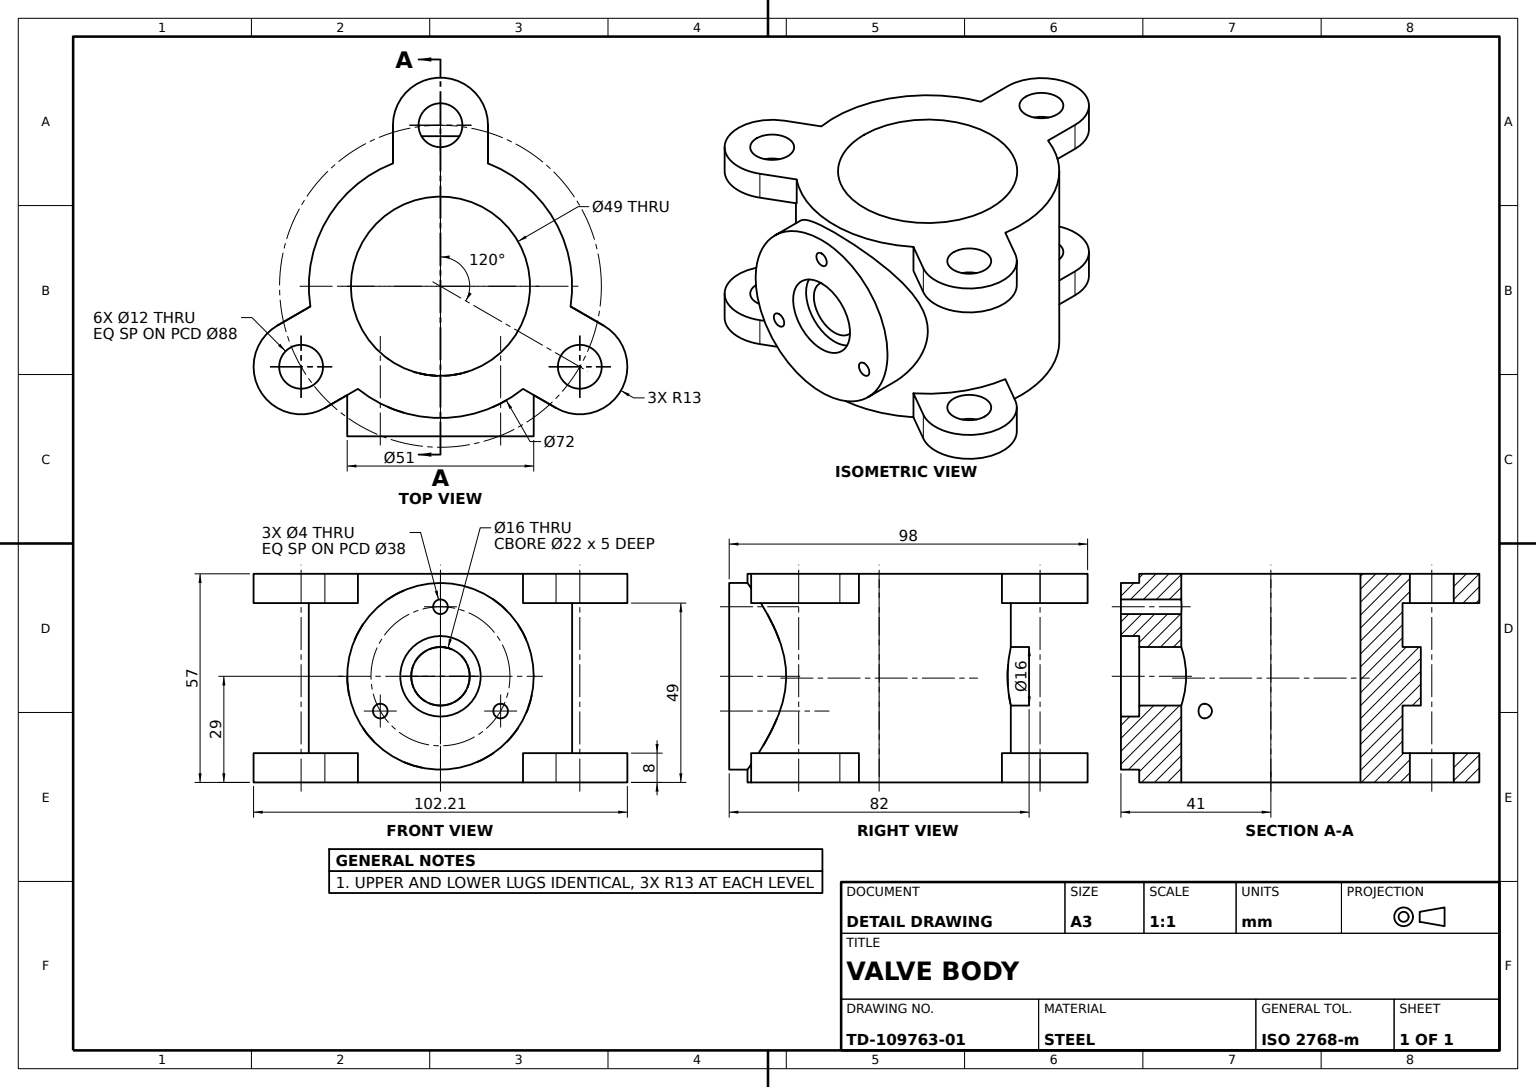
ISO-10303-21;
HEADER;
FILE_DESCRIPTION((''),'2;1');
FILE_NAME('','',(''),(''),'','','');
FILE_SCHEMA(('AUTOMOTIVE_DESIGN'));
ENDSEC;
DATA;
#1=APPLICATION_CONTEXT('');
#2=PRODUCT_CONTEXT('',#1,'mechanical');
#3=PRODUCT('','','',(#2));
#4=PRODUCT_DEFINITION_FORMATION('','',#3);
#5=PRODUCT_DEFINITION_CONTEXT('',#1,'design');
#6=PRODUCT_DEFINITION('','',#4,#5);
#7=PRODUCT_DEFINITION_SHAPE('','',#6);
#8=(LENGTH_UNIT()NAMED_UNIT(*)SI_UNIT(.MILLI.,.METRE.));
#9=(NAMED_UNIT(*)PLANE_ANGLE_UNIT()SI_UNIT($,.RADIAN.));
#10=(NAMED_UNIT(*)SI_UNIT($,.STERADIAN.)SOLID_ANGLE_UNIT());
#11=UNCERTAINTY_MEASURE_WITH_UNIT(LENGTH_MEASURE(0.005),#8,'distance_accuracy_value','');
#12=(GEOMETRIC_REPRESENTATION_CONTEXT(3)GLOBAL_UNCERTAINTY_ASSIGNED_CONTEXT((#11))GLOBAL_UNIT_ASSIGNED_CONTEXT((#8,#9,#10))REPRESENTATION_CONTEXT('',''));
#13=CARTESIAN_POINT('',(-13.,44.,8.));
#14=VERTEX_POINT('',#13);
#15=CARTESIAN_POINT('',(-13.,44.,0.));
#16=VERTEX_POINT('',#15);
#17=DIRECTION('',(0.,0.,-1.));
#18=VECTOR('',#17,1000.);
#19=LINE('',#13,#18);
#20=EDGE_CURVE('',#14,#16,#19,.T.);
#21=ORIENTED_EDGE('',*,*,#20,.T.);
#22=CARTESIAN_POINT('',(-13.,33.570821,0.));
#23=VERTEX_POINT('',#22);
#24=DIRECTION('',(0.,-1.,0.));
#25=VECTOR('',#24,1000.);
#26=LINE('',#15,#25);
#27=EDGE_CURVE('',#16,#23,#26,.T.);
#28=ORIENTED_EDGE('',*,*,#27,.T.);
#29=CARTESIAN_POINT('',(-13.,33.570821,8.));
#30=VERTEX_POINT('',#29);
#31=CARTESIAN_POINT('',(-13.,33.570821,57.));
#32=LINE('',#31,#18);
#33=EDGE_CURVE('',#30,#23,#32,.T.);
#34=ORIENTED_EDGE('',*,*,#33,.F.);
#35=LINE('',#13,#25);
#36=EDGE_CURVE('',#14,#30,#35,.T.);
#37=ORIENTED_EDGE('',*,*,#36,.F.);
#38=EDGE_LOOP('',(#21,#28,#34,#37));
#39=FACE_BOUND('',#38,.T.);
#40=DIRECTION('',(1.,0.,0.));
#41=DIRECTION('',(0.,1.,0.));
#42=AXIS2_PLACEMENT_3D('',#13,#40,#41);
#43=PLANE('',#42);
#44=ADVANCED_FACE('',(#39),#43,.F.);
#45=CARTESIAN_POINT('',(13.,44.,8.));
#46=VERTEX_POINT('',#45);
#47=CARTESIAN_POINT('',(0.,44.,8.));
#48=DIRECTION('',(0.,0.,1.));
#49=AXIS2_PLACEMENT_3D('',#47,#48,#40);
#50=CIRCLE('',#49,13.);
#51=EDGE_CURVE('',#46,#14,#50,.T.);
#52=ORIENTED_EDGE('',*,*,#51,.T.);
#53=ORIENTED_EDGE('',*,*,#36,.T.);
#54=CARTESIAN_POINT('',(13.,33.570821,8.));
#55=VERTEX_POINT('',#54);
#56=CARTESIAN_POINT('',(0.,0.,8.));
#57=AXIS2_PLACEMENT_3D('',#56,#48,#40);
#58=CIRCLE('',#57,36.);
#59=EDGE_CURVE('',#30,#55,#58,.F.);
#60=ORIENTED_EDGE('',*,*,#59,.T.);
#61=CARTESIAN_POINT('',(13.,19.247574,8.));
#62=VECTOR('',#41,1000.);
#63=LINE('',#61,#62);
#64=EDGE_CURVE('',#55,#46,#63,.T.);
#65=ORIENTED_EDGE('',*,*,#64,.T.);
#66=EDGE_LOOP('',(#52,#53,#60,#65));
#67=FACE_BOUND('',#66,.T.);
#68=CARTESIAN_POINT('',(-6.,44.,8.));
#69=VERTEX_POINT('',#68);
#70=DIRECTION('',(-1.,0.,0.));
#71=AXIS2_PLACEMENT_3D('',#47,#17,#70);
#72=CIRCLE('',#71,6.);
#73=EDGE_CURVE('',#69,#69,#72,.T.);
#74=ORIENTED_EDGE('',*,*,#73,.T.);
#75=EDGE_LOOP('',(#74));
#76=FACE_BOUND('',#75,.T.);
#77=PLANE('',#49);
#78=ADVANCED_FACE('',(#67,#76),#77,.T.);
#79=CARTESIAN_POINT('',(0.,-41.,40.));
#80=VERTEX_POINT('',#79);
#81=CARTESIAN_POINT('',(0.,-41.,29.));
#82=AXIS2_PLACEMENT_3D('',#81,#41,#48);
#83=CIRCLE('',#82,11.);
#84=EDGE_CURVE('',#80,#80,#83,.T.);
#85=ORIENTED_EDGE('',*,*,#84,.F.);
#86=EDGE_LOOP('',(#85));
#87=FACE_BOUND('',#86,.T.);
#88=CARTESIAN_POINT('',(0.,-36.,40.));
#89=VERTEX_POINT('',#88);
#90=CARTESIAN_POINT('',(0.,-36.,29.));
#91=AXIS2_PLACEMENT_3D('',#90,#41,#48);
#92=CIRCLE('',#91,11.);
#93=EDGE_CURVE('',#89,#89,#92,.F.);
#94=ORIENTED_EDGE('',*,*,#93,.F.);
#95=EDGE_LOOP('',(#94));
#96=FACE_BOUND('',#95,.T.);
#97=CYLINDRICAL_SURFACE('',#82,11.);
#98=ADVANCED_FACE('',(#87,#96),#97,.F.);
#99=CARTESIAN_POINT('',(-31.605118,-33.25833,57.));
#100=VERTEX_POINT('',#99);
#101=CARTESIAN_POINT('',(-31.605118,-33.25833,49.));
#102=VERTEX_POINT('',#101);
#103=LINE('',#99,#18);
#104=EDGE_CURVE('',#100,#102,#103,.T.);
#105=ORIENTED_EDGE('',*,*,#104,.T.);
#106=CARTESIAN_POINT('',(-22.573184,-28.043741,49.));
#107=VERTEX_POINT('',#106);
#108=DIRECTION('',(0.866025404,0.5,0.));
#109=VECTOR('',#108,1000.);
#110=LINE('',#101,#109);
#111=EDGE_CURVE('',#102,#107,#110,.T.);
#112=ORIENTED_EDGE('',*,*,#111,.T.);
#113=CARTESIAN_POINT('',(-22.573184,-28.043741,57.));
#114=VERTEX_POINT('',#113);
#115=LINE('',#113,#18);
#116=EDGE_CURVE('',#114,#107,#115,.T.);
#117=ORIENTED_EDGE('',*,*,#116,.F.);
#118=LINE('',#99,#109);
#119=EDGE_CURVE('',#100,#114,#118,.T.);
#120=ORIENTED_EDGE('',*,*,#119,.F.);
#121=EDGE_LOOP('',(#105,#112,#117,#120));
#122=FACE_BOUND('',#121,.T.);
#123=DIRECTION('',(-0.5,0.866025404,0.));
#124=DIRECTION('',(-0.866025404,-0.5,0.));
#125=AXIS2_PLACEMENT_3D('',#99,#123,#124);
#126=PLANE('',#125);
#127=ADVANCED_FACE('',(#122),#126,.F.);
#128=CARTESIAN_POINT('',(8.,41.,29.));
#129=VERTEX_POINT('',#128);
#130=CARTESIAN_POINT('',(0.,41.,29.));
#131=AXIS2_PLACEMENT_3D('',#130,#24,#40);
#132=CIRCLE('',#131,8.);
#133=EDGE_CURVE('',#129,#129,#132,.T.);
#134=ORIENTED_EDGE('',*,*,#133,.F.);
#135=EDGE_LOOP('',(#134));
#136=FACE_BOUND('',#135,.T.);
#137=AXIS2_PLACEMENT_3D('',#130,#24,#17);
#138=PLANE('',#137);
#139=ADVANCED_FACE('',(#136),#138,.F.);
#140=CARTESIAN_POINT('',(0.,-24.5,50.));
#141=VERTEX_POINT('',#140);
#142=CARTESIAN_POINT('',(1.568988,-24.45908,49.565975));
#143=CARTESIAN_POINT('',(-0.000396,-24.52044,50.216889));
#144=CARTESIAN_POINT('',(-1.567404,-24.459158,49.566467));
#145=CARTESIAN_POINT('',(-2.216103,-24.397775,48.001691));
#146=CARTESIAN_POINT('',(-1.568183,-24.459126,46.433265));
#147=CARTESIAN_POINT('',(-0.000356,-24.520392,45.783879));
#148=CARTESIAN_POINT('',(1.565251,-24.459308,46.431221));
#149=CARTESIAN_POINT('',(2.216439,-24.39775,47.997771));
#150=B_SPLINE_CURVE_WITH_KNOTS('',3,(#142,#143,#144,#145,#146,#147,#148,#149,#142,#143,#144),.UNSPECIFIED.,.T.,.F.,(1,1,1,1,1,1,1,1,1,1,1,1,1,1,1),(-0.004691091,-0.003127394,-0.001563697,0.,0.001563697,0.003127394,0.004691091,0.006254789,0.007818486,0.009382183,0.01094588,0.012509577,0.014073274,0.015636972,0.017200669),.UNSPECIFIED.);
#151=EDGE_CURVE('',#141,#141,#150,.T.);
#152=ORIENTED_EDGE('',*,*,#151,.F.);
#153=EDGE_LOOP('',(#152));
#154=FACE_BOUND('',#153,.T.);
#155=CARTESIAN_POINT('',(0.,-41.,50.));
#156=VERTEX_POINT('',#155);
#157=CARTESIAN_POINT('',(0.,-41.,48.));
#158=AXIS2_PLACEMENT_3D('',#157,#41,#48);
#159=CIRCLE('',#158,2.);
#160=EDGE_CURVE('',#156,#156,#159,.T.);
#161=ORIENTED_EDGE('',*,*,#160,.F.);
#162=EDGE_LOOP('',(#161));
#163=FACE_BOUND('',#162,.T.);
#164=CYLINDRICAL_SURFACE('',#158,2.);
#165=ADVANCED_FACE('',(#154,#163),#164,.F.);
#166=CARTESIAN_POINT('',(25.5,-41.,29.));
#167=VERTEX_POINT('',#166);
#168=AXIS2_PLACEMENT_3D('',#81,#24,#40);
#169=CIRCLE('',#168,25.5);
#170=EDGE_CURVE('',#167,#167,#169,.T.);
#171=ORIENTED_EDGE('',*,*,#170,.F.);
#172=EDGE_LOOP('',(#171));
#173=FACE_BOUND('',#172,.T.);
#174=CARTESIAN_POINT('',(0.,-36.,54.5));
#175=VERTEX_POINT('',#174);
#176=CARTESIAN_POINT('',(-2.623968,-35.935367,54.408867));
#177=CARTESIAN_POINT('',(0.00209,-36.032249,54.545468));
#178=CARTESIAN_POINT('',(2.615608,-35.935638,54.409262));
#179=CARTESIAN_POINT('',(6.004809,-35.567496,53.887383));
#180=CARTESIAN_POINT('',(9.302281,-34.841941,52.846053));
#181=CARTESIAN_POINT('',(12.282274,-33.866344,51.393122));
#182=CARTESIAN_POINT('',(15.110257,-32.735138,49.655989));
#183=CARTESIAN_POINT('',(18.206348,-31.140232,47.071248));
#184=CARTESIAN_POINT('',(21.285882,-29.097399,43.312835));
#185=CARTESIAN_POINT('',(23.206509,-27.543877,39.792813));
#186=CARTESIAN_POINT('',(24.37095,-26.503081,36.645505));
#187=CARTESIAN_POINT('',(25.009127,-25.898094,34.191474));
#188=CARTESIAN_POINT('',(25.407874,-25.504561,31.64284));
#189=CARTESIAN_POINT('',(25.544396,-25.366798,29.008017));
#190=CARTESIAN_POINT('',(25.414507,-25.497952,26.430217));
#191=CARTESIAN_POINT('',(24.886386,-26.019293,22.989721));
#192=CARTESIAN_POINT('',(23.632329,-27.197946,19.003808));
#193=CARTESIAN_POINT('',(21.283753,-29.098179,14.682968));
#194=CARTESIAN_POINT('',(18.770232,-30.769502,11.608265));
#195=CARTESIAN_POINT('',(16.376156,-32.082651,9.402489));
#196=CARTESIAN_POINT('',(13.80026,-33.304629,7.451454));
#197=CARTESIAN_POINT('',(10.928245,-34.369027,5.851187));
#198=CARTESIAN_POINT('',(7.723412,-35.19114,4.653079));
#199=CARTESIAN_POINT('',(4.434427,-35.796635,3.785689));
#200=CARTESIAN_POINT('',(0.920616,-36.061872,3.412957));
#201=CARTESIAN_POINT('',(-2.525487,-35.942391,3.58115));
#202=CARTESIAN_POINT('',(-5.975113,-35.573987,4.103445));
#203=CARTESIAN_POINT('',(-10.049777,-34.682644,5.381776));
#204=CARTESIAN_POINT('',(-13.723079,-33.338264,7.399303));
#205=CARTESIAN_POINT('',(-16.314869,-32.11383,9.351586));
#206=CARTESIAN_POINT('',(-18.719175,-30.801086,11.552633));
#207=CARTESIAN_POINT('',(-21.249753,-29.123757,14.630907));
#208=CARTESIAN_POINT('',(-23.220037,-27.532642,18.23707));
#209=CARTESIAN_POINT('',(-24.365105,-26.508337,21.3385));
#210=CARTESIAN_POINT('',(-25.22676,-25.691389,24.6396));
#211=CARTESIAN_POINT('',(-25.590222,-25.319942,28.095515));
#212=CARTESIAN_POINT('',(-25.410398,-25.502111,31.613837));
#213=CARTESIAN_POINT('',(-24.885882,-26.019948,35.005302));
#214=CARTESIAN_POINT('',(-23.609674,-27.217252,39.052827));
#215=CARTESIAN_POINT('',(-21.278045,-29.103558,43.326155));
#216=CARTESIAN_POINT('',(-18.721276,-30.798812,46.443468));
#217=CARTESIAN_POINT('',(-16.347608,-32.097442,48.62155));
#218=CARTESIAN_POINT('',(-13.7232,-33.337955,50.600597));
#219=CARTESIAN_POINT('',(-10.151487,-34.651526,52.572014));
#220=CARTESIAN_POINT('',(-6.026689,-35.56441,53.883076));
#221=B_SPLINE_CURVE_WITH_KNOTS('',3,(#176,#177,#178,#179,#180,#181,#182,#183,#184,#185,#186,#187,#188,#189,#190,#191,#192,#193,#194,#195,#196,#197,#198,#199,#200,#201,#202,#203,#204,#205,#206,#207,#208,#209,#210,#211,#212,#213,#214,#215,#216,#217,#218,#219,#220,#176,#177,#178),.UNSPECIFIED.,.T.,.F.,(1,1,1,1,1,1,1,1,1,1,1,1,1,1,1,1,1,1,1,1,1,1,1,1,1,1,1,1,1,1,1,1,1,1,1,1,1,1,1,1,1,1,1,1,1,1,1,1,1,1,1,1),(-0.01036361,-0.005181805,-0.002590903,0.,0.002590903,0.005181805,0.01036361,0.012954513,0.015545416,0.020727221,0.025909026,0.031090831,0.033681734,0.036272637,0.038863539,0.041454442,0.044045344,0.046636247,0.051818052,0.056999858,0.062181663,0.064772565,0.067363468,0.072545273,0.075136176,0.077727078,0.082908884,0.085499786,0.088090689,0.093272494,0.098454299,0.101045202,0.103636105,0.10881791,0.113999715,0.116590618,0.11918152,0.124363326,0.126954228,0.129545131,0.134726936,0.139908741,0.145090547,0.147681449,0.150272352,0.155454157,0.160635962,0.163226865,0.165817767,0.16840867,0.170999573,0.176181378),.UNSPECIFIED.);
#222=EDGE_CURVE('',#175,#175,#221,.T.);
#223=ORIENTED_EDGE('',*,*,#222,.F.);
#224=EDGE_LOOP('',(#223));
#225=FACE_BOUND('',#224,.T.);
#226=CYLINDRICAL_SURFACE('',#82,25.5);
#227=ADVANCED_FACE('',(#173,#225),#226,.T.);
#228=CARTESIAN_POINT('',(-35.573184,-5.52708,0.));
#229=VERTEX_POINT('',#228);
#230=CARTESIAN_POINT('',(-35.573184,-5.52708,8.));
#231=VERTEX_POINT('',#230);
#232=CARTESIAN_POINT('',(-35.573184,-5.52708,57.));
#233=LINE('',#232,#18);
#234=EDGE_CURVE('',#229,#231,#233,.F.);
#235=ORIENTED_EDGE('',*,*,#234,.F.);
#236=CARTESIAN_POINT('',(-44.605118,-10.74167,0.));
#237=VERTEX_POINT('',#236);
#238=CARTESIAN_POINT('',(-23.168888,1.634543,0.));
#239=VECTOR('',#124,1000.);
#240=LINE('',#238,#239);
#241=EDGE_CURVE('',#229,#237,#240,.T.);
#242=ORIENTED_EDGE('',*,*,#241,.T.);
#243=CARTESIAN_POINT('',(-44.605118,-10.74167,8.));
#244=VERTEX_POINT('',#243);
#245=LINE('',#243,#18);
#246=EDGE_CURVE('',#244,#237,#245,.T.);
#247=ORIENTED_EDGE('',*,*,#246,.F.);
#248=CARTESIAN_POINT('',(-23.168888,1.634543,8.));
#249=LINE('',#248,#239);
#250=EDGE_CURVE('',#231,#244,#249,.T.);
#251=ORIENTED_EDGE('',*,*,#250,.F.);
#252=EDGE_LOOP('',(#235,#242,#247,#251));
#253=FACE_BOUND('',#252,.T.);
#254=DIRECTION('',(0.5,-0.866025404,0.));
#255=AXIS2_PLACEMENT_3D('',#248,#254,#108);
#256=PLANE('',#255);
#257=ADVANCED_FACE('',(#253),#256,.F.);
#258=CARTESIAN_POINT('',(-44.105118,-22.,57.));
#259=VERTEX_POINT('',#258);
#260=CARTESIAN_POINT('',(-38.105118,-22.,57.));
#261=AXIS2_PLACEMENT_3D('',#260,#17,#70);
#262=CIRCLE('',#261,6.);
#263=EDGE_CURVE('',#259,#259,#262,.T.);
#264=ORIENTED_EDGE('',*,*,#263,.F.);
#265=EDGE_LOOP('',(#264));
#266=FACE_BOUND('',#265,.T.);
#267=CARTESIAN_POINT('',(-32.105118,-22.,49.));
#268=VERTEX_POINT('',#267);
#269=CARTESIAN_POINT('',(-38.105118,-22.,49.));
#270=AXIS2_PLACEMENT_3D('',#269,#48,#40);
#271=CIRCLE('',#270,6.);
#272=EDGE_CURVE('',#268,#268,#271,.T.);
#273=ORIENTED_EDGE('',*,*,#272,.F.);
#274=EDGE_LOOP('',(#273));
#275=FACE_BOUND('',#274,.T.);
#276=CYLINDRICAL_SURFACE('',#261,6.);
#277=ADVANCED_FACE('',(#266,#275),#276,.F.);
#278=CARTESIAN_POINT('',(-44.605118,-10.74167,49.));
#279=VERTEX_POINT('',#278);
#280=AXIS2_PLACEMENT_3D('',#269,#48,#123);
#281=CIRCLE('',#280,13.);
#282=EDGE_CURVE('',#279,#102,#281,.T.);
#283=ORIENTED_EDGE('',*,*,#282,.F.);
#284=CARTESIAN_POINT('',(-35.573184,-5.52708,49.));
#285=VERTEX_POINT('',#284);
#286=CARTESIAN_POINT('',(-23.168888,1.634543,49.));
#287=LINE('',#286,#239);
#288=EDGE_CURVE('',#285,#279,#287,.T.);
#289=ORIENTED_EDGE('',*,*,#288,.F.);
#290=CARTESIAN_POINT('',(0.,0.,49.));
#291=AXIS2_PLACEMENT_3D('',#290,#48,#40);
#292=CIRCLE('',#291,36.);
#293=EDGE_CURVE('',#107,#285,#292,.F.);
#294=ORIENTED_EDGE('',*,*,#293,.F.);
#295=ORIENTED_EDGE('',*,*,#111,.F.);
#296=EDGE_LOOP('',(#283,#289,#294,#295));
#297=FACE_BOUND('',#296,.T.);
#298=ORIENTED_EDGE('',*,*,#272,.T.);
#299=EDGE_LOOP('',(#298));
#300=FACE_BOUND('',#299,.T.);
#301=PLANE('',#270);
#302=ADVANCED_FACE('',(#297,#300),#301,.F.);
#303=CARTESIAN_POINT('',(44.605118,-10.74167,57.));
#304=VERTEX_POINT('',#303);
#305=CARTESIAN_POINT('',(44.605118,-10.74167,49.));
#306=VERTEX_POINT('',#305);
#307=LINE('',#303,#18);
#308=EDGE_CURVE('',#304,#306,#307,.T.);
#309=ORIENTED_EDGE('',*,*,#308,.T.);
#310=CARTESIAN_POINT('',(35.573184,-5.52708,49.));
#311=VERTEX_POINT('',#310);
#312=DIRECTION('',(-0.866025404,0.5,0.));
#313=VECTOR('',#312,1000.);
#314=LINE('',#305,#313);
#315=EDGE_CURVE('',#306,#311,#314,.T.);
#316=ORIENTED_EDGE('',*,*,#315,.T.);
#317=CARTESIAN_POINT('',(35.573184,-5.52708,57.));
#318=VERTEX_POINT('',#317);
#319=LINE('',#317,#18);
#320=EDGE_CURVE('',#318,#311,#319,.T.);
#321=ORIENTED_EDGE('',*,*,#320,.F.);
#322=LINE('',#303,#313);
#323=EDGE_CURVE('',#304,#318,#322,.T.);
#324=ORIENTED_EDGE('',*,*,#323,.F.);
#325=EDGE_LOOP('',(#309,#316,#321,#324));
#326=FACE_BOUND('',#325,.T.);
#327=DIRECTION('',(-0.5,-0.866025404,0.));
#328=DIRECTION('',(0.866025404,-0.5,0.));
#329=AXIS2_PLACEMENT_3D('',#303,#327,#328);
#330=PLANE('',#329);
#331=ADVANCED_FACE('',(#326),#330,.F.);
#332=CARTESIAN_POINT('',(44.105118,-22.,8.));
#333=VERTEX_POINT('',#332);
#334=CARTESIAN_POINT('',(38.105118,-22.,8.));
#335=AXIS2_PLACEMENT_3D('',#334,#48,#40);
#336=CIRCLE('',#335,6.);
#337=EDGE_CURVE('',#333,#333,#336,.T.);
#338=ORIENTED_EDGE('',*,*,#337,.F.);
#339=EDGE_LOOP('',(#338));
#340=FACE_BOUND('',#339,.T.);
#341=CARTESIAN_POINT('',(44.605118,-10.74167,8.));
#342=VERTEX_POINT('',#341);
#343=CARTESIAN_POINT('',(35.573184,-5.52708,8.));
#344=VERTEX_POINT('',#343);
#345=LINE('',#341,#313);
#346=EDGE_CURVE('',#342,#344,#345,.T.);
#347=ORIENTED_EDGE('',*,*,#346,.T.);
#348=CARTESIAN_POINT('',(22.573184,-28.043741,8.));
#349=VERTEX_POINT('',#348);
#350=EDGE_CURVE('',#344,#349,#58,.F.);
#351=ORIENTED_EDGE('',*,*,#350,.T.);
#352=CARTESIAN_POINT('',(31.605118,-33.25833,8.));
#353=VERTEX_POINT('',#352);
#354=CARTESIAN_POINT('',(10.168888,-20.882117,8.));
#355=VECTOR('',#328,1000.);
#356=LINE('',#354,#355);
#357=EDGE_CURVE('',#349,#353,#356,.T.);
#358=ORIENTED_EDGE('',*,*,#357,.T.);
#359=AXIS2_PLACEMENT_3D('',#334,#48,#327);
#360=CIRCLE('',#359,13.);
#361=EDGE_CURVE('',#353,#342,#360,.T.);
#362=ORIENTED_EDGE('',*,*,#361,.T.);
#363=EDGE_LOOP('',(#347,#351,#358,#362));
#364=FACE_BOUND('',#363,.T.);
#365=PLANE('',#335);
#366=ADVANCED_FACE('',(#340,#364),#365,.T.);
#367=CARTESIAN_POINT('',(-16.454483,-41.,21.5));
#368=VERTEX_POINT('',#367);
#369=CARTESIAN_POINT('',(-16.454483,-41.,19.5));
#370=AXIS2_PLACEMENT_3D('',#369,#41,#48);
#371=CIRCLE('',#370,2.);
#372=EDGE_CURVE('',#368,#368,#371,.T.);
#373=ORIENTED_EDGE('',*,*,#372,.F.);
#374=EDGE_LOOP('',(#373));
#375=FACE_BOUND('',#374,.T.);
#376=CARTESIAN_POINT('',(-16.454483,-18.152135,21.5));
#377=VERTEX_POINT('',#376);
#378=CARTESIAN_POINT('',(-15.262742,-19.177495,21.265406));
#379=CARTESIAN_POINT('',(-16.237822,-18.365662,21.577732));
#380=CARTESIAN_POINT('',(-17.131574,-17.522123,21.422617));
#381=CARTESIAN_POINT('',(-17.745543,-16.899065,21.082093));
#382=CARTESIAN_POINT('',(-18.25071,-16.348867,20.504695));
#383=CARTESIAN_POINT('',(-18.529005,-16.028671,19.61639));
#384=CARTESIAN_POINT('',(-18.343226,-16.243768,18.667117));
#385=CARTESIAN_POINT('',(-17.871596,-16.765256,18.027668));
#386=CARTESIAN_POINT('',(-17.279763,-17.375803,17.635356));
#387=CARTESIAN_POINT('',(-16.395357,-18.225034,17.412327));
#388=CARTESIAN_POINT('',(-15.425953,-19.047731,17.644373));
#389=CARTESIAN_POINT('',(-14.659831,-19.632499,18.476299));
#390=CARTESIAN_POINT('',(-14.381879,-19.834343,19.38135));
#391=CARTESIAN_POINT('',(-14.558131,-19.707092,20.330723));
#392=B_SPLINE_CURVE_WITH_KNOTS('',3,(#378,#379,#380,#381,#382,#383,#384,#385,#386,#387,#388,#389,#390,#391,#378,#379,#380),.UNSPECIFIED.,.T.,.F.,(1,1,1,1,1,1,1,1,1,1,1,1,1,1,1,1,1,1,1,1,1),(-0.003692806,-0.002769605,-0.001846403,0.,0.000923202,0.001846403,0.002769605,0.003692806,0.004616008,0.005539209,0.006462411,0.007385612,0.009232016,0.010155217,0.011078419,0.01200162,0.012924822,0.014771225,0.015694427,0.016617628,0.01754083),.UNSPECIFIED.);
#393=EDGE_CURVE('',#377,#377,#392,.T.);
#394=ORIENTED_EDGE('',*,*,#393,.F.);
#395=EDGE_LOOP('',(#394));
#396=FACE_BOUND('',#395,.T.);
#397=CYLINDRICAL_SURFACE('',#370,2.);
#398=ADVANCED_FACE('',(#375,#396),#397,.F.);
#399=CARTESIAN_POINT('',(44.105118,-22.,49.));
#400=VERTEX_POINT('',#399);
#401=CARTESIAN_POINT('',(38.105118,-22.,49.));
#402=AXIS2_PLACEMENT_3D('',#401,#48,#40);
#403=CIRCLE('',#402,6.);
#404=EDGE_CURVE('',#400,#400,#403,.T.);
#405=ORIENTED_EDGE('',*,*,#404,.T.);
#406=EDGE_LOOP('',(#405));
#407=FACE_BOUND('',#406,.T.);
#408=ORIENTED_EDGE('',*,*,#315,.F.);
#409=CARTESIAN_POINT('',(31.605118,-33.25833,49.));
#410=VERTEX_POINT('',#409);
#411=AXIS2_PLACEMENT_3D('',#401,#48,#327);
#412=CIRCLE('',#411,13.);
#413=EDGE_CURVE('',#410,#306,#412,.T.);
#414=ORIENTED_EDGE('',*,*,#413,.F.);
#415=CARTESIAN_POINT('',(22.573184,-28.043741,49.));
#416=VERTEX_POINT('',#415);
#417=CARTESIAN_POINT('',(10.168888,-20.882117,49.));
#418=LINE('',#417,#355);
#419=EDGE_CURVE('',#416,#410,#418,.T.);
#420=ORIENTED_EDGE('',*,*,#419,.F.);
#421=EDGE_CURVE('',#311,#416,#292,.F.);
#422=ORIENTED_EDGE('',*,*,#421,.F.);
#423=EDGE_LOOP('',(#408,#414,#420,#422));
#424=FACE_BOUND('',#423,.T.);
#425=PLANE('',#402);
#426=ADVANCED_FACE('',(#407,#424),#425,.F.);
#427=ORIENTED_EDGE('',*,*,#133,.T.);
#428=EDGE_LOOP('',(#427));
#429=FACE_BOUND('',#428,.T.);
#430=CARTESIAN_POINT('',(0.,36.,21.));
#431=VERTEX_POINT('',#430);
#432=CARTESIAN_POINT('',(3.161828,35.902254,21.424462));
#433=CARTESIAN_POINT('',(-0.002449,36.048709,20.788534));
#434=CARTESIAN_POINT('',(-3.152031,35.902911,21.421403));
#435=CARTESIAN_POINT('',(-5.804069,35.553263,23.198652));
#436=CARTESIAN_POINT('',(-7.578557,35.199789,25.848603));
#437=CARTESIAN_POINT('',(-8.209745,35.050099,28.994317));
#438=CARTESIAN_POINT('',(-7.582453,35.198962,32.14483));
#439=CARTESIAN_POINT('',(-5.803491,35.553425,34.802824));
#440=CARTESIAN_POINT('',(-3.150422,35.903097,36.579286));
#441=CARTESIAN_POINT('',(-0.003507,36.048314,37.209709));
#442=CARTESIAN_POINT('',(3.144568,35.903644,36.581872));
#443=CARTESIAN_POINT('',(5.798008,35.554304,34.807374));
#444=CARTESIAN_POINT('',(7.576893,35.200203,32.157368));
#445=CARTESIAN_POINT('',(8.210398,35.049934,29.004799));
#446=CARTESIAN_POINT('',(7.581507,35.199208,25.853728));
#447=CARTESIAN_POINT('',(5.805573,35.552826,23.201301));
#448=B_SPLINE_CURVE_WITH_KNOTS('',3,(#432,#433,#434,#435,#436,#437,#438,#439,#440,#441,#442,#443,#444,#445,#446,#447,#432,#433,#434),.UNSPECIFIED.,.T.,.F.,(1,1,1,1,1,1,1,1,1,1,1,1,1,1,1,1,1,1,1,1,1,1,1),(-0.009407565,-0.00627171,-0.003135855,0.,0.003135855,0.00627171,0.009407565,0.01254342,0.015679275,0.01881513,0.021950985,0.02508684,0.028222695,0.03135855,0.034494405,0.037630261,0.040766116,0.043901971,0.047037826,0.050173681,0.053309536,0.056445391,0.059581246),.UNSPECIFIED.);
#449=EDGE_CURVE('',#431,#431,#448,.T.);
#450=ORIENTED_EDGE('',*,*,#449,.T.);
#451=EDGE_LOOP('',(#450));
#452=FACE_BOUND('',#451,.T.);
#453=CYLINDRICAL_SURFACE('',#137,8.);
#454=ADVANCED_FACE('',(#429,#452),#453,.T.);
#455=CARTESIAN_POINT('',(13.,33.570821,57.));
#456=VERTEX_POINT('',#455);
#457=CARTESIAN_POINT('',(13.,44.,57.));
#458=VERTEX_POINT('',#457);
#459=CARTESIAN_POINT('',(13.,19.247574,57.));
#460=LINE('',#459,#62);
#461=EDGE_CURVE('',#456,#458,#460,.T.);
#462=ORIENTED_EDGE('',*,*,#461,.T.);
#463=CARTESIAN_POINT('',(-13.,44.,57.));
#464=VERTEX_POINT('',#463);
#465=CARTESIAN_POINT('',(0.,44.,57.));
#466=AXIS2_PLACEMENT_3D('',#465,#48,#40);
#467=CIRCLE('',#466,13.);
#468=EDGE_CURVE('',#458,#464,#467,.T.);
#469=ORIENTED_EDGE('',*,*,#468,.T.);
#470=VERTEX_POINT('',#31);
#471=LINE('',#463,#25);
#472=EDGE_CURVE('',#464,#470,#471,.T.);
#473=ORIENTED_EDGE('',*,*,#472,.T.);
#474=VERTEX_POINT('',#232);
#475=CARTESIAN_POINT('',(0.,0.,57.));
#476=AXIS2_PLACEMENT_3D('',#475,#17,#40);
#477=CIRCLE('',#476,36.);
#478=EDGE_CURVE('',#474,#470,#477,.T.);
#479=ORIENTED_EDGE('',*,*,#478,.F.);
#480=CARTESIAN_POINT('',(-44.605118,-10.74167,57.));
#481=VERTEX_POINT('',#480);
#482=CARTESIAN_POINT('',(-23.168888,1.634543,57.));
#483=LINE('',#482,#239);
#484=EDGE_CURVE('',#474,#481,#483,.T.);
#485=ORIENTED_EDGE('',*,*,#484,.T.);
#486=AXIS2_PLACEMENT_3D('',#260,#48,#123);
#487=CIRCLE('',#486,13.);
#488=EDGE_CURVE('',#481,#100,#487,.T.);
#489=ORIENTED_EDGE('',*,*,#488,.T.);
#490=ORIENTED_EDGE('',*,*,#119,.T.);
#491=CARTESIAN_POINT('',(22.573184,-28.043741,57.));
#492=VERTEX_POINT('',#491);
#493=EDGE_CURVE('',#492,#114,#477,.T.);
#494=ORIENTED_EDGE('',*,*,#493,.F.);
#495=CARTESIAN_POINT('',(31.605118,-33.25833,57.));
#496=VERTEX_POINT('',#495);
#497=CARTESIAN_POINT('',(10.168888,-20.882117,57.));
#498=LINE('',#497,#355);
#499=EDGE_CURVE('',#492,#496,#498,.T.);
#500=ORIENTED_EDGE('',*,*,#499,.T.);
#501=CARTESIAN_POINT('',(38.105118,-22.,57.));
#502=AXIS2_PLACEMENT_3D('',#501,#48,#327);
#503=CIRCLE('',#502,13.);
#504=EDGE_CURVE('',#496,#304,#503,.T.);
#505=ORIENTED_EDGE('',*,*,#504,.T.);
#506=ORIENTED_EDGE('',*,*,#323,.T.);
#507=EDGE_CURVE('',#456,#318,#477,.T.);
#508=ORIENTED_EDGE('',*,*,#507,.F.);
#509=EDGE_LOOP('',(#462,#469,#473,#479,#485,#489,#490,#494,#500,#505,#506,#508));
#510=FACE_BOUND('',#509,.T.);
#511=ORIENTED_EDGE('',*,*,#263,.T.);
#512=EDGE_LOOP('',(#511));
#513=FACE_BOUND('',#512,.T.);
#514=CARTESIAN_POINT('',(-6.,44.,57.));
#515=VERTEX_POINT('',#514);
#516=AXIS2_PLACEMENT_3D('',#465,#17,#70);
#517=CIRCLE('',#516,6.);
#518=EDGE_CURVE('',#515,#515,#517,.T.);
#519=ORIENTED_EDGE('',*,*,#518,.T.);
#520=EDGE_LOOP('',(#519));
#521=FACE_BOUND('',#520,.T.);
#522=CARTESIAN_POINT('',(-24.5,0.,57.));
#523=VERTEX_POINT('',#522);
#524=AXIS2_PLACEMENT_3D('',#475,#17,#70);
#525=CIRCLE('',#524,24.5);
#526=EDGE_CURVE('',#523,#523,#525,.T.);
#527=ORIENTED_EDGE('',*,*,#526,.T.);
#528=EDGE_LOOP('',(#527));
#529=FACE_BOUND('',#528,.T.);
#530=CARTESIAN_POINT('',(32.105118,-22.,57.));
#531=VERTEX_POINT('',#530);
#532=AXIS2_PLACEMENT_3D('',#501,#17,#70);
#533=CIRCLE('',#532,6.);
#534=EDGE_CURVE('',#531,#531,#533,.T.);
#535=ORIENTED_EDGE('',*,*,#534,.T.);
#536=EDGE_LOOP('',(#535));
#537=FACE_BOUND('',#536,.T.);
#538=PLANE('',#524);
#539=ADVANCED_FACE('',(#510,#513,#521,#529,#537),#538,.F.);
#540=CARTESIAN_POINT('',(13.,44.,49.));
#541=VERTEX_POINT('',#540);
#542=CARTESIAN_POINT('',(-13.,44.,49.));
#543=VERTEX_POINT('',#542);
#544=CARTESIAN_POINT('',(0.,44.,49.));
#545=AXIS2_PLACEMENT_3D('',#544,#48,#40);
#546=CIRCLE('',#545,13.);
#547=EDGE_CURVE('',#541,#543,#546,.T.);
#548=ORIENTED_EDGE('',*,*,#547,.T.);
#549=LINE('',#463,#18);
#550=EDGE_CURVE('',#464,#543,#549,.T.);
#551=ORIENTED_EDGE('',*,*,#550,.F.);
#552=ORIENTED_EDGE('',*,*,#468,.F.);
#553=LINE('',#457,#18);
#554=EDGE_CURVE('',#458,#541,#553,.T.);
#555=ORIENTED_EDGE('',*,*,#554,.T.);
#556=EDGE_LOOP('',(#548,#551,#552,#555));
#557=FACE_BOUND('',#556,.T.);
#558=CYLINDRICAL_SURFACE('',#516,13.);
#559=ADVANCED_FACE('',(#557),#558,.T.);
#560=CARTESIAN_POINT('',(32.105118,-22.,0.));
#561=VERTEX_POINT('',#560);
#562=CARTESIAN_POINT('',(38.105118,-22.,0.));
#563=AXIS2_PLACEMENT_3D('',#562,#17,#70);
#564=CIRCLE('',#563,6.);
#565=EDGE_CURVE('',#561,#561,#564,.T.);
#566=ORIENTED_EDGE('',*,*,#565,.T.);
#567=EDGE_LOOP('',(#566));
#568=FACE_BOUND('',#567,.T.);
#569=ORIENTED_EDGE('',*,*,#337,.T.);
#570=EDGE_LOOP('',(#569));
#571=FACE_BOUND('',#570,.T.);
#572=CYLINDRICAL_SURFACE('',#532,6.);
#573=ADVANCED_FACE('',(#568,#571),#572,.F.);
#574=ORIENTED_EDGE('',*,*,#404,.F.);
#575=EDGE_LOOP('',(#574));
#576=FACE_BOUND('',#575,.T.);
#577=ORIENTED_EDGE('',*,*,#534,.F.);
#578=EDGE_LOOP('',(#577));
#579=FACE_BOUND('',#578,.T.);
#580=ADVANCED_FACE('',(#576,#579),#572,.F.);
#581=CARTESIAN_POINT('',(16.454483,-41.,21.5));
#582=VERTEX_POINT('',#581);
#583=CARTESIAN_POINT('',(16.454483,-41.,19.5));
#584=AXIS2_PLACEMENT_3D('',#583,#41,#48);
#585=CIRCLE('',#584,2.);
#586=EDGE_CURVE('',#582,#582,#585,.T.);
#587=ORIENTED_EDGE('',*,*,#586,.F.);
#588=EDGE_LOOP('',(#587));
#589=FACE_BOUND('',#588,.T.);
#590=CARTESIAN_POINT('',(16.454483,-18.152135,21.5));
#591=VERTEX_POINT('',#590);
#592=CARTESIAN_POINT('',(17.135699,-17.518168,21.421622));
#593=CARTESIAN_POINT('',(16.23492,-18.368378,21.578124));
#594=CARTESIAN_POINT('',(15.266559,-19.174301,21.266643));
#595=CARTESIAN_POINT('',(14.562485,-19.703924,20.33781));
#596=CARTESIAN_POINT('',(14.381153,-19.834854,19.398071));
#597=CARTESIAN_POINT('',(14.654108,-19.63675,18.484075));
#598=CARTESIAN_POINT('',(15.421172,-19.051618,17.646623));
#599=CARTESIAN_POINT('',(16.389351,-18.230415,17.412603));
#600=CARTESIAN_POINT('',(17.274574,-17.38099,17.633022));
#601=CARTESIAN_POINT('',(17.867921,-16.769204,18.023972));
#602=CARTESIAN_POINT('',(18.341111,-16.246193,18.66281));
#603=CARTESIAN_POINT('',(18.529549,-16.028037,19.610093));
#604=CARTESIAN_POINT('',(18.252286,-16.347101,20.502602));
#605=CARTESIAN_POINT('',(17.747903,-16.896527,21.079736));
#606=B_SPLINE_CURVE_WITH_KNOTS('',3,(#592,#593,#594,#595,#596,#597,#598,#599,#600,#601,#602,#603,#604,#605,#592,#593,#594),.UNSPECIFIED.,.T.,.F.,(1,1,1,1,1,1,1,1,1,1,1,1,1,1,1,1,1,1,1,1,1),(-0.002777255,-0.001851503,-0.000925752,0.,0.001851503,0.002777255,0.003703006,0.004628758,0.005554509,0.007406012,0.008331764,0.009257516,0.010183267,0.011109019,0.01203477,0.012960522,0.013886273,0.014812025,0.016663528,0.01758928,0.018515031),.UNSPECIFIED.);
#607=EDGE_CURVE('',#591,#591,#606,.T.);
#608=ORIENTED_EDGE('',*,*,#607,.F.);
#609=EDGE_LOOP('',(#608));
#610=FACE_BOUND('',#609,.T.);
#611=CYLINDRICAL_SURFACE('',#584,2.);
#612=ADVANCED_FACE('',(#589,#610),#611,.F.);
#613=ORIENTED_EDGE('',*,*,#507,.T.);
#614=ORIENTED_EDGE('',*,*,#320,.T.);
#615=ORIENTED_EDGE('',*,*,#421,.T.);
#616=LINE('',#491,#18);
#617=EDGE_CURVE('',#416,#492,#616,.F.);
#618=ORIENTED_EDGE('',*,*,#617,.T.);
#619=ORIENTED_EDGE('',*,*,#493,.T.);
#620=ORIENTED_EDGE('',*,*,#116,.T.);
#621=ORIENTED_EDGE('',*,*,#293,.T.);
#622=EDGE_CURVE('',#285,#474,#233,.F.);
#623=ORIENTED_EDGE('',*,*,#622,.T.);
#624=ORIENTED_EDGE('',*,*,#478,.T.);
#625=CARTESIAN_POINT('',(-13.,33.570821,49.));
#626=VERTEX_POINT('',#625);
#627=EDGE_CURVE('',#470,#626,#32,.T.);
#628=ORIENTED_EDGE('',*,*,#627,.T.);
#629=CARTESIAN_POINT('',(13.,33.570821,49.));
#630=VERTEX_POINT('',#629);
#631=EDGE_CURVE('',#626,#630,#292,.F.);
#632=ORIENTED_EDGE('',*,*,#631,.T.);
#633=LINE('',#455,#18);
#634=EDGE_CURVE('',#630,#456,#633,.F.);
#635=ORIENTED_EDGE('',*,*,#634,.T.);
#636=EDGE_LOOP('',(#613,#614,#615,#618,#619,#620,#621,#623,#624,#628,#632,#635));
#637=FACE_BOUND('',#636,.T.);
#638=ORIENTED_EDGE('',*,*,#449,.F.);
#639=EDGE_LOOP('',(#638));
#640=FACE_BOUND('',#639,.T.);
#641=ORIENTED_EDGE('',*,*,#350,.F.);
#642=CARTESIAN_POINT('',(35.573184,-5.52708,0.));
#643=VERTEX_POINT('',#642);
#644=EDGE_CURVE('',#344,#643,#319,.T.);
#645=ORIENTED_EDGE('',*,*,#644,.T.);
#646=CARTESIAN_POINT('',(13.,33.570821,0.));
#647=VERTEX_POINT('',#646);
#648=CARTESIAN_POINT('',(0.,0.,0.));
#649=AXIS2_PLACEMENT_3D('',#648,#17,#40);
#650=CIRCLE('',#649,36.);
#651=EDGE_CURVE('',#647,#643,#650,.T.);
#652=ORIENTED_EDGE('',*,*,#651,.F.);
#653=EDGE_CURVE('',#647,#55,#633,.F.);
#654=ORIENTED_EDGE('',*,*,#653,.T.);
#655=ORIENTED_EDGE('',*,*,#59,.F.);
#656=ORIENTED_EDGE('',*,*,#33,.T.);
#657=EDGE_CURVE('',#229,#23,#650,.T.);
#658=ORIENTED_EDGE('',*,*,#657,.F.);
#659=ORIENTED_EDGE('',*,*,#234,.T.);
#660=CARTESIAN_POINT('',(-22.573184,-28.043741,8.));
#661=VERTEX_POINT('',#660);
#662=EDGE_CURVE('',#661,#231,#58,.F.);
#663=ORIENTED_EDGE('',*,*,#662,.F.);
#664=CARTESIAN_POINT('',(-22.573184,-28.043741,0.));
#665=VERTEX_POINT('',#664);
#666=EDGE_CURVE('',#661,#665,#115,.T.);
#667=ORIENTED_EDGE('',*,*,#666,.T.);
#668=CARTESIAN_POINT('',(22.573184,-28.043741,0.));
#669=VERTEX_POINT('',#668);
#670=EDGE_CURVE('',#669,#665,#650,.T.);
#671=ORIENTED_EDGE('',*,*,#670,.F.);
#672=EDGE_CURVE('',#669,#349,#616,.F.);
#673=ORIENTED_EDGE('',*,*,#672,.T.);
#674=EDGE_LOOP('',(#641,#645,#652,#654,#655,#656,#658,#659,#663,#667,#671,#673));
#675=FACE_BOUND('',#674,.T.);
#676=ORIENTED_EDGE('',*,*,#222,.T.);
#677=EDGE_LOOP('',(#676));
#678=FACE_BOUND('',#677,.T.);
#679=CYLINDRICAL_SURFACE('',#524,36.);
#680=ADVANCED_FACE('',(#637,#640,#675,#678),#679,.T.);
#681=CARTESIAN_POINT('',(31.605118,-33.25833,0.));
#682=VERTEX_POINT('',#681);
#683=LINE('',#352,#18);
#684=EDGE_CURVE('',#353,#682,#683,.T.);
#685=ORIENTED_EDGE('',*,*,#684,.T.);
#686=CARTESIAN_POINT('',(44.605118,-10.74167,0.));
#687=VERTEX_POINT('',#686);
#688=AXIS2_PLACEMENT_3D('',#562,#48,#327);
#689=CIRCLE('',#688,13.);
#690=EDGE_CURVE('',#682,#687,#689,.T.);
#691=ORIENTED_EDGE('',*,*,#690,.T.);
#692=LINE('',#341,#18);
#693=EDGE_CURVE('',#342,#687,#692,.T.);
#694=ORIENTED_EDGE('',*,*,#693,.F.);
#695=ORIENTED_EDGE('',*,*,#361,.F.);
#696=EDGE_LOOP('',(#685,#691,#694,#695));
#697=FACE_BOUND('',#696,.T.);
#698=AXIS2_PLACEMENT_3D('',#334,#17,#70);
#699=CYLINDRICAL_SURFACE('',#698,13.);
#700=ADVANCED_FACE('',(#697),#699,.T.);
#701=CARTESIAN_POINT('',(0.,-36.,37.));
#702=VERTEX_POINT('',#701);
#703=CIRCLE('',#91,8.);
#704=EDGE_CURVE('',#702,#702,#703,.F.);
#705=ORIENTED_EDGE('',*,*,#704,.F.);
#706=EDGE_LOOP('',(#705));
#707=FACE_BOUND('',#706,.T.);
#708=ORIENTED_EDGE('',*,*,#93,.T.);
#709=EDGE_LOOP('',(#708));
#710=FACE_BOUND('',#709,.T.);
#711=PLANE('',#91);
#712=ADVANCED_FACE('',(#707,#710),#711,.F.);
#713=ORIENTED_EDGE('',*,*,#104,.F.);
#714=ORIENTED_EDGE('',*,*,#488,.F.);
#715=LINE('',#480,#18);
#716=EDGE_CURVE('',#481,#279,#715,.T.);
#717=ORIENTED_EDGE('',*,*,#716,.T.);
#718=ORIENTED_EDGE('',*,*,#282,.T.);
#719=EDGE_LOOP('',(#713,#714,#717,#718));
#720=FACE_BOUND('',#719,.T.);
#721=CYLINDRICAL_SURFACE('',#261,13.);
#722=ADVANCED_FACE('',(#720),#721,.T.);
#723=CARTESIAN_POINT('',(13.,44.,0.));
#724=VERTEX_POINT('',#723);
#725=CARTESIAN_POINT('',(13.,19.247574,0.));
#726=LINE('',#725,#62);
#727=EDGE_CURVE('',#647,#724,#726,.T.);
#728=ORIENTED_EDGE('',*,*,#727,.T.);
#729=LINE('',#45,#18);
#730=EDGE_CURVE('',#46,#724,#729,.T.);
#731=ORIENTED_EDGE('',*,*,#730,.F.);
#732=ORIENTED_EDGE('',*,*,#64,.F.);
#733=ORIENTED_EDGE('',*,*,#653,.F.);
#734=EDGE_LOOP('',(#728,#731,#732,#733));
#735=FACE_BOUND('',#734,.T.);
#736=AXIS2_PLACEMENT_3D('',#61,#70,#24);
#737=PLANE('',#736);
#738=ADVANCED_FACE('',(#735),#737,.F.);
#739=CARTESIAN_POINT('',(0.,44.,0.));
#740=AXIS2_PLACEMENT_3D('',#739,#48,#40);
#741=CIRCLE('',#740,13.);
#742=EDGE_CURVE('',#724,#16,#741,.T.);
#743=ORIENTED_EDGE('',*,*,#742,.T.);
#744=ORIENTED_EDGE('',*,*,#20,.F.);
#745=ORIENTED_EDGE('',*,*,#51,.F.);
#746=ORIENTED_EDGE('',*,*,#730,.T.);
#747=EDGE_LOOP('',(#743,#744,#745,#746));
#748=FACE_BOUND('',#747,.T.);
#749=CYLINDRICAL_SURFACE('',#71,13.);
#750=ADVANCED_FACE('',(#748),#749,.T.);
#751=ORIENTED_EDGE('',*,*,#84,.T.);
#752=EDGE_LOOP('',(#751));
#753=FACE_BOUND('',#752,.T.);
#754=ORIENTED_EDGE('',*,*,#160,.T.);
#755=EDGE_LOOP('',(#754));
#756=FACE_BOUND('',#755,.T.);
#757=ORIENTED_EDGE('',*,*,#170,.T.);
#758=EDGE_LOOP('',(#757));
#759=FACE_BOUND('',#758,.T.);
#760=ORIENTED_EDGE('',*,*,#372,.T.);
#761=EDGE_LOOP('',(#760));
#762=FACE_BOUND('',#761,.T.);
#763=ORIENTED_EDGE('',*,*,#586,.T.);
#764=EDGE_LOOP('',(#763));
#765=FACE_BOUND('',#764,.T.);
#766=AXIS2_PLACEMENT_3D('',#81,#24,#17);
#767=PLANE('',#766);
#768=ADVANCED_FACE('',(#753,#756,#759,#762,#765),#767,.T.);
#769=CARTESIAN_POINT('',(6.,44.,49.));
#770=VERTEX_POINT('',#769);
#771=CIRCLE('',#545,6.);
#772=EDGE_CURVE('',#770,#770,#771,.T.);
#773=ORIENTED_EDGE('',*,*,#772,.T.);
#774=EDGE_LOOP('',(#773));
#775=FACE_BOUND('',#774,.T.);
#776=CARTESIAN_POINT('',(13.,19.247574,49.));
#777=LINE('',#776,#62);
#778=EDGE_CURVE('',#630,#541,#777,.T.);
#779=ORIENTED_EDGE('',*,*,#778,.F.);
#780=ORIENTED_EDGE('',*,*,#631,.F.);
#781=LINE('',#542,#25);
#782=EDGE_CURVE('',#543,#626,#781,.T.);
#783=ORIENTED_EDGE('',*,*,#782,.F.);
#784=ORIENTED_EDGE('',*,*,#547,.F.);
#785=EDGE_LOOP('',(#779,#780,#783,#784));
#786=FACE_BOUND('',#785,.T.);
#787=PLANE('',#545);
#788=ADVANCED_FACE('',(#775,#786),#787,.F.);
#789=ORIENTED_EDGE('',*,*,#672,.F.);
#790=CARTESIAN_POINT('',(10.168888,-20.882117,0.));
#791=LINE('',#790,#355);
#792=EDGE_CURVE('',#669,#682,#791,.T.);
#793=ORIENTED_EDGE('',*,*,#792,.T.);
#794=ORIENTED_EDGE('',*,*,#684,.F.);
#795=ORIENTED_EDGE('',*,*,#357,.F.);
#796=EDGE_LOOP('',(#789,#793,#794,#795));
#797=FACE_BOUND('',#796,.T.);
#798=DIRECTION('',(0.5,0.866025404,0.));
#799=AXIS2_PLACEMENT_3D('',#354,#798,#312);
#800=PLANE('',#799);
#801=ADVANCED_FACE('',(#797),#800,.F.);
#802=ORIENTED_EDGE('',*,*,#151,.T.);
#803=EDGE_LOOP('',(#802));
#804=FACE_BOUND('',#803,.T.);
#805=CARTESIAN_POINT('',(0.,-24.5,37.));
#806=VERTEX_POINT('',#805);
#807=CARTESIAN_POINT('',(3.165921,-24.355936,36.573387));
#808=CARTESIAN_POINT('',(-0.000533,-24.571967,37.213088));
#809=CARTESIAN_POINT('',(-3.16379,-24.356194,36.57426));
#810=CARTESIAN_POINT('',(-5.803662,-23.839645,34.798475));
#811=CARTESIAN_POINT('',(-7.57391,-23.31053,32.16174));
#812=CARTESIAN_POINT('',(-8.212105,-23.080637,29.00719));
#813=CARTESIAN_POINT('',(-7.577661,-23.309359,25.84271));
#814=CARTESIAN_POINT('',(-5.800262,-23.84066,23.197234));
#815=CARTESIAN_POINT('',(-3.160218,-24.356493,21.425029));
#816=CARTESIAN_POINT('',(-0.003931,-24.571567,20.788099));
#817=CARTESIAN_POINT('',(3.156381,-24.357239,21.422581));
#818=CARTESIAN_POINT('',(5.800713,-23.84055,23.197557));
#819=CARTESIAN_POINT('',(7.575366,-23.310078,25.839538));
#820=CARTESIAN_POINT('',(8.212171,-23.08061,28.998737));
#821=CARTESIAN_POINT('',(7.57595,-23.309914,32.15933));
#822=CARTESIAN_POINT('',(5.802627,-23.839862,34.799288));
#823=B_SPLINE_CURVE_WITH_KNOTS('',3,(#807,#808,#809,#810,#811,#812,#813,#814,#815,#816,#817,#818,#819,#820,#821,#822,#807,#808,#809),.UNSPECIFIED.,.T.,.F.,(1,1,1,1,1,1,1,1,1,1,1,1,1,1,1,1,1,1,1,1,1,1,1),(-0.009443364,-0.006295576,-0.003147788,0.,0.003147788,0.006295576,0.009443364,0.012591152,0.01573894,0.018886728,0.022034516,0.025182304,0.028330092,0.03147788,0.034625668,0.037773456,0.040921244,0.044069032,0.04721682,0.050364608,0.053512396,0.056660184,0.059807972),.UNSPECIFIED.);
#824=EDGE_CURVE('',#806,#806,#823,.T.);
#825=ORIENTED_EDGE('',*,*,#824,.T.);
#826=EDGE_LOOP('',(#825));
#827=FACE_BOUND('',#826,.T.);
#828=CARTESIAN_POINT('',(-24.5,0.,0.));
#829=VERTEX_POINT('',#828);
#830=AXIS2_PLACEMENT_3D('',#648,#17,#70);
#831=CIRCLE('',#830,24.5);
#832=EDGE_CURVE('',#829,#829,#831,.T.);
#833=ORIENTED_EDGE('',*,*,#832,.T.);
#834=EDGE_LOOP('',(#833));
#835=FACE_BOUND('',#834,.T.);
#836=ORIENTED_EDGE('',*,*,#526,.F.);
#837=EDGE_LOOP('',(#836));
#838=FACE_BOUND('',#837,.T.);
#839=ORIENTED_EDGE('',*,*,#607,.T.);
#840=EDGE_LOOP('',(#839));
#841=FACE_BOUND('',#840,.T.);
#842=ORIENTED_EDGE('',*,*,#393,.T.);
#843=EDGE_LOOP('',(#842));
#844=FACE_BOUND('',#843,.T.);
#845=CYLINDRICAL_SURFACE('',#524,24.5);
#846=ADVANCED_FACE('',(#804,#827,#835,#838,#841,#844),#845,.F.);
#847=CARTESIAN_POINT('',(-6.,44.,0.));
#848=VERTEX_POINT('',#847);
#849=AXIS2_PLACEMENT_3D('',#739,#17,#70);
#850=CIRCLE('',#849,6.);
#851=EDGE_CURVE('',#848,#848,#850,.T.);
#852=ORIENTED_EDGE('',*,*,#851,.F.);
#853=EDGE_LOOP('',(#852));
#854=FACE_BOUND('',#853,.T.);
#855=ORIENTED_EDGE('',*,*,#565,.F.);
#856=EDGE_LOOP('',(#855));
#857=FACE_BOUND('',#856,.T.);
#858=ORIENTED_EDGE('',*,*,#832,.F.);
#859=EDGE_LOOP('',(#858));
#860=FACE_BOUND('',#859,.T.);
#861=CARTESIAN_POINT('',(-44.105118,-22.,0.));
#862=VERTEX_POINT('',#861);
#863=CARTESIAN_POINT('',(-38.105118,-22.,0.));
#864=AXIS2_PLACEMENT_3D('',#863,#17,#70);
#865=CIRCLE('',#864,6.);
#866=EDGE_CURVE('',#862,#862,#865,.T.);
#867=ORIENTED_EDGE('',*,*,#866,.F.);
#868=EDGE_LOOP('',(#867));
#869=FACE_BOUND('',#868,.T.);
#870=ORIENTED_EDGE('',*,*,#651,.T.);
#871=LINE('',#686,#313);
#872=EDGE_CURVE('',#687,#643,#871,.T.);
#873=ORIENTED_EDGE('',*,*,#872,.F.);
#874=ORIENTED_EDGE('',*,*,#690,.F.);
#875=ORIENTED_EDGE('',*,*,#792,.F.);
#876=ORIENTED_EDGE('',*,*,#670,.T.);
#877=CARTESIAN_POINT('',(-31.605118,-33.25833,0.));
#878=VERTEX_POINT('',#877);
#879=LINE('',#877,#109);
#880=EDGE_CURVE('',#878,#665,#879,.T.);
#881=ORIENTED_EDGE('',*,*,#880,.F.);
#882=AXIS2_PLACEMENT_3D('',#863,#48,#123);
#883=CIRCLE('',#882,13.);
#884=EDGE_CURVE('',#237,#878,#883,.T.);
#885=ORIENTED_EDGE('',*,*,#884,.F.);
#886=ORIENTED_EDGE('',*,*,#241,.F.);
#887=ORIENTED_EDGE('',*,*,#657,.T.);
#888=ORIENTED_EDGE('',*,*,#27,.F.);
#889=ORIENTED_EDGE('',*,*,#742,.F.);
#890=ORIENTED_EDGE('',*,*,#727,.F.);
#891=EDGE_LOOP('',(#870,#873,#874,#875,#876,#881,#885,#886,#887,#888,#889,#890));
#892=FACE_BOUND('',#891,.T.);
#893=PLANE('',#830);
#894=ADVANCED_FACE('',(#854,#857,#860,#869,#892),#893,.T.);
#895=ORIENTED_EDGE('',*,*,#461,.F.);
#896=ORIENTED_EDGE('',*,*,#634,.F.);
#897=ORIENTED_EDGE('',*,*,#778,.T.);
#898=ORIENTED_EDGE('',*,*,#554,.F.);
#899=EDGE_LOOP('',(#895,#896,#897,#898));
#900=FACE_BOUND('',#899,.T.);
#901=AXIS2_PLACEMENT_3D('',#459,#70,#24);
#902=PLANE('',#901);
#903=ADVANCED_FACE('',(#900),#902,.F.);
#904=ORIENTED_EDGE('',*,*,#413,.T.);
#905=ORIENTED_EDGE('',*,*,#308,.F.);
#906=ORIENTED_EDGE('',*,*,#504,.F.);
#907=LINE('',#495,#18);
#908=EDGE_CURVE('',#496,#410,#907,.T.);
#909=ORIENTED_EDGE('',*,*,#908,.T.);
#910=EDGE_LOOP('',(#904,#905,#906,#909));
#911=FACE_BOUND('',#910,.T.);
#912=CYLINDRICAL_SURFACE('',#532,13.);
#913=ADVANCED_FACE('',(#911),#912,.T.);
#914=ORIENTED_EDGE('',*,*,#346,.F.);
#915=ORIENTED_EDGE('',*,*,#693,.T.);
#916=ORIENTED_EDGE('',*,*,#872,.T.);
#917=ORIENTED_EDGE('',*,*,#644,.F.);
#918=EDGE_LOOP('',(#914,#915,#916,#917));
#919=FACE_BOUND('',#918,.T.);
#920=AXIS2_PLACEMENT_3D('',#341,#327,#328);
#921=PLANE('',#920);
#922=ADVANCED_FACE('',(#919),#921,.F.);
#923=ORIENTED_EDGE('',*,*,#866,.T.);
#924=EDGE_LOOP('',(#923));
#925=FACE_BOUND('',#924,.T.);
#926=CARTESIAN_POINT('',(-32.105118,-22.,8.));
#927=VERTEX_POINT('',#926);
#928=CARTESIAN_POINT('',(-38.105118,-22.,8.));
#929=AXIS2_PLACEMENT_3D('',#928,#48,#40);
#930=CIRCLE('',#929,6.);
#931=EDGE_CURVE('',#927,#927,#930,.T.);
#932=ORIENTED_EDGE('',*,*,#931,.T.);
#933=EDGE_LOOP('',(#932));
#934=FACE_BOUND('',#933,.T.);
#935=ADVANCED_FACE('',(#925,#934),#276,.F.);
#936=ORIENTED_EDGE('',*,*,#782,.T.);
#937=ORIENTED_EDGE('',*,*,#627,.F.);
#938=ORIENTED_EDGE('',*,*,#472,.F.);
#939=ORIENTED_EDGE('',*,*,#550,.T.);
#940=EDGE_LOOP('',(#936,#937,#938,#939));
#941=FACE_BOUND('',#940,.T.);
#942=AXIS2_PLACEMENT_3D('',#463,#40,#41);
#943=PLANE('',#942);
#944=ADVANCED_FACE('',(#941),#943,.F.);
#945=ORIENTED_EDGE('',*,*,#419,.T.);
#946=ORIENTED_EDGE('',*,*,#908,.F.);
#947=ORIENTED_EDGE('',*,*,#499,.F.);
#948=ORIENTED_EDGE('',*,*,#617,.F.);
#949=EDGE_LOOP('',(#945,#946,#947,#948));
#950=FACE_BOUND('',#949,.T.);
#951=AXIS2_PLACEMENT_3D('',#497,#798,#312);
#952=PLANE('',#951);
#953=ADVANCED_FACE('',(#950),#952,.F.);
#954=ORIENTED_EDGE('',*,*,#484,.F.);
#955=ORIENTED_EDGE('',*,*,#622,.F.);
#956=ORIENTED_EDGE('',*,*,#288,.T.);
#957=ORIENTED_EDGE('',*,*,#716,.F.);
#958=EDGE_LOOP('',(#954,#955,#956,#957));
#959=FACE_BOUND('',#958,.T.);
#960=AXIS2_PLACEMENT_3D('',#482,#254,#108);
#961=PLANE('',#960);
#962=ADVANCED_FACE('',(#959),#961,.F.);
#963=CARTESIAN_POINT('',(-31.605118,-33.25833,8.));
#964=VERTEX_POINT('',#963);
#965=AXIS2_PLACEMENT_3D('',#928,#48,#123);
#966=CIRCLE('',#965,13.);
#967=EDGE_CURVE('',#244,#964,#966,.T.);
#968=ORIENTED_EDGE('',*,*,#967,.T.);
#969=LINE('',#963,#109);
#970=EDGE_CURVE('',#964,#661,#969,.T.);
#971=ORIENTED_EDGE('',*,*,#970,.T.);
#972=ORIENTED_EDGE('',*,*,#662,.T.);
#973=ORIENTED_EDGE('',*,*,#250,.T.);
#974=EDGE_LOOP('',(#968,#971,#972,#973));
#975=FACE_BOUND('',#974,.T.);
#976=ORIENTED_EDGE('',*,*,#931,.F.);
#977=EDGE_LOOP('',(#976));
#978=FACE_BOUND('',#977,.T.);
#979=PLANE('',#929);
#980=ADVANCED_FACE('',(#975,#978),#979,.T.);
#981=ORIENTED_EDGE('',*,*,#704,.T.);
#982=EDGE_LOOP('',(#981));
#983=FACE_BOUND('',#982,.T.);
#984=ORIENTED_EDGE('',*,*,#824,.F.);
#985=EDGE_LOOP('',(#984));
#986=FACE_BOUND('',#985,.T.);
#987=CARTESIAN_POINT('',(0.,9.,29.));
#988=AXIS2_PLACEMENT_3D('',#987,#41,#48);
#989=CYLINDRICAL_SURFACE('',#988,8.);
#990=ADVANCED_FACE('',(#983,#986),#989,.F.);
#991=ORIENTED_EDGE('',*,*,#666,.F.);
#992=ORIENTED_EDGE('',*,*,#970,.F.);
#993=LINE('',#963,#18);
#994=EDGE_CURVE('',#964,#878,#993,.T.);
#995=ORIENTED_EDGE('',*,*,#994,.T.);
#996=ORIENTED_EDGE('',*,*,#880,.T.);
#997=EDGE_LOOP('',(#991,#992,#995,#996));
#998=FACE_BOUND('',#997,.T.);
#999=AXIS2_PLACEMENT_3D('',#963,#123,#124);
#1000=PLANE('',#999);
#1001=ADVANCED_FACE('',(#998),#1000,.F.);
#1002=ORIENTED_EDGE('',*,*,#73,.F.);
#1003=EDGE_LOOP('',(#1002));
#1004=FACE_BOUND('',#1003,.T.);
#1005=ORIENTED_EDGE('',*,*,#851,.T.);
#1006=EDGE_LOOP('',(#1005));
#1007=FACE_BOUND('',#1006,.T.);
#1008=CYLINDRICAL_SURFACE('',#71,6.);
#1009=ADVANCED_FACE('',(#1004,#1007),#1008,.F.);
#1010=ORIENTED_EDGE('',*,*,#518,.F.);
#1011=EDGE_LOOP('',(#1010));
#1012=FACE_BOUND('',#1011,.T.);
#1013=ORIENTED_EDGE('',*,*,#772,.F.);
#1014=EDGE_LOOP('',(#1013));
#1015=FACE_BOUND('',#1014,.T.);
#1016=CYLINDRICAL_SURFACE('',#545,6.);
#1017=ADVANCED_FACE('',(#1012,#1015),#1016,.F.);
#1018=ORIENTED_EDGE('',*,*,#884,.T.);
#1019=ORIENTED_EDGE('',*,*,#994,.F.);
#1020=ORIENTED_EDGE('',*,*,#967,.F.);
#1021=ORIENTED_EDGE('',*,*,#246,.T.);
#1022=EDGE_LOOP('',(#1018,#1019,#1020,#1021));
#1023=FACE_BOUND('',#1022,.T.);
#1024=AXIS2_PLACEMENT_3D('',#928,#17,#70);
#1025=CYLINDRICAL_SURFACE('',#1024,13.);
#1026=ADVANCED_FACE('',(#1023),#1025,.T.);
#1027=CLOSED_SHELL('',(#44,#78,#98,#127,#139,#165,#227,#257,#277,#302,#331,#366,#398,#426,#454,#539,#559,#573,#580,#612,#680,#700,#712,#722,#738,#750,#768,#788,#801,#846,#894,#903,#913,#922,#935,#944,#953,#962,#980,#990,#1001,#1009,#1017,#1026));
#1028=MANIFOLD_SOLID_BREP('',#1027);
#1029=ADVANCED_BREP_SHAPE_REPRESENTATION('',(#1028),#12);
#1030=SHAPE_DEFINITION_REPRESENTATION(#7,#1029);
ENDSEC;
END-ISO-10303-21;
